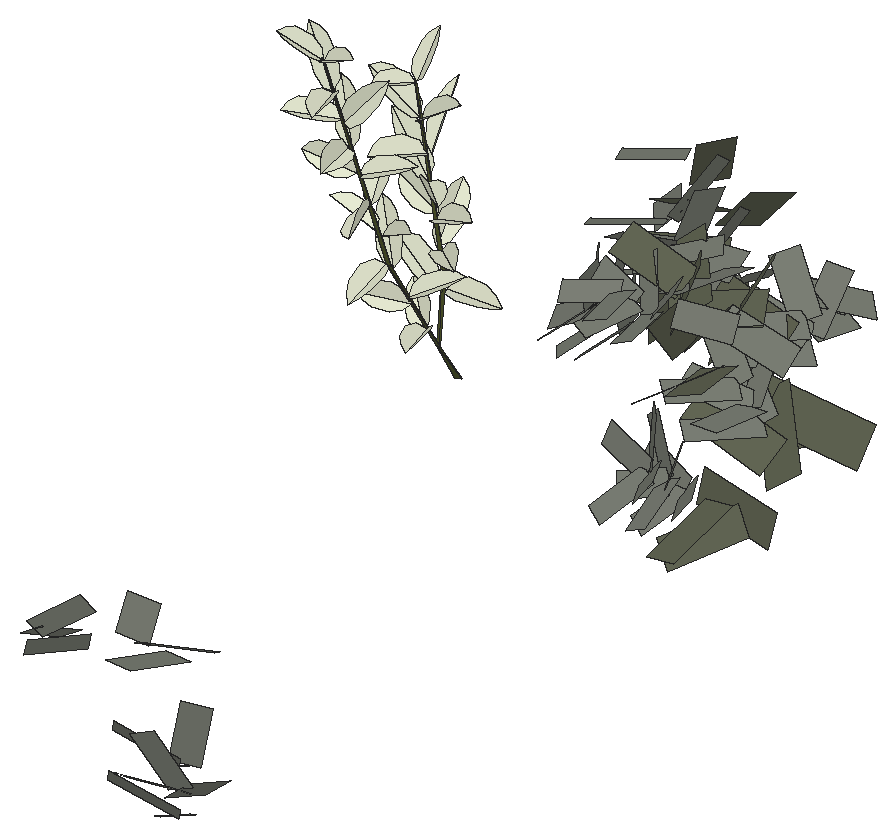
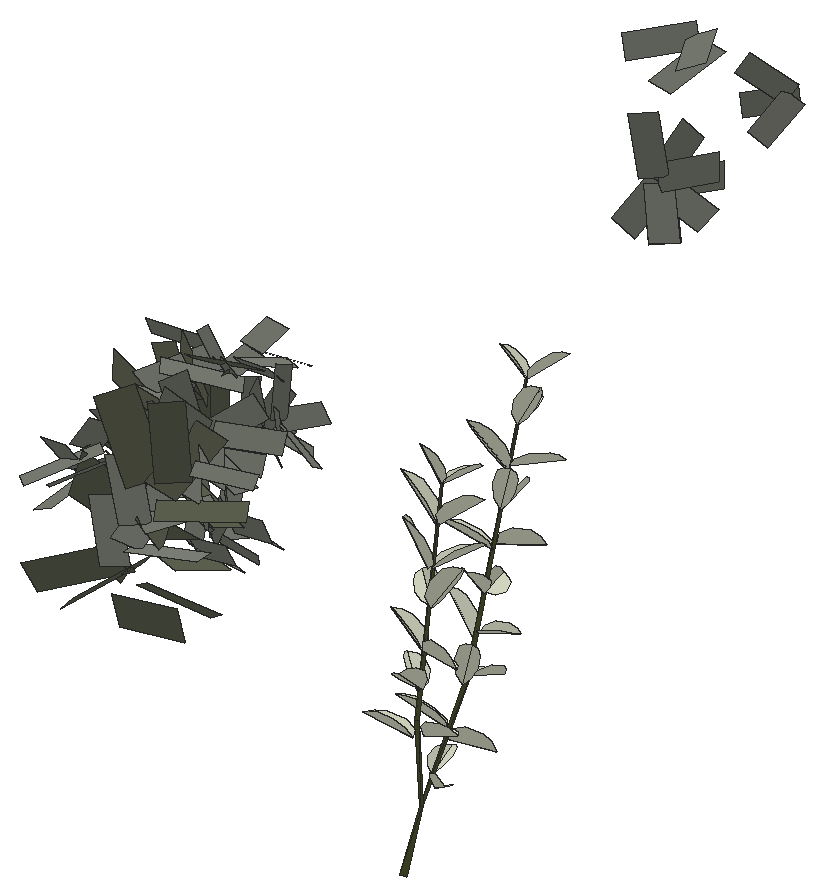
# SketchUp Ruby script. Lengths in inches.
U = 1.inch
M = Sketchup.active_model
def pt(a) = Geom::Point3d.new(a.map { |v| v * U })
def face(e, loops, mat)
  f = e.add_face(loops[0].map { |a| pt(a) })
  loops[1..].each { |l| e.add_face(l.map { |a| pt(a) }).erase! }
  f.material = f.back_material = mat if mat
  f
end
# faces: each face lists its corners as indices into pts; further lists are holes
def faces(e, pts, list, mat = nil) = list.each { |f| face(e, (f[0].is_a?(Array) ? f : [f]).map { |l| l.map { |i| pts[i] } }, mat) }
# xy, xz, yz: faces in a plane at the given z, y or x. An outline is a flat list of corners, or four numbers for a rectangle; further outlines are holes
def ring(l) = l.size == 4 ? [[l[0], l[1]], [l[2], l[1]], [l[2], l[3]], [l[0], l[3]]] : l.each_slice(2).to_a
def flat(e, list, mat, &to3) = list.each { |f| face(e, (f[0].is_a?(Array) ? f : [f]).map { |l| ring(l).map { |u, v| to3.(u, v) } }, mat) }
def xy(e, z, list, mat = nil) = flat(e, list, mat) { |x, y| [x, y, z] }
def xz(e, y, list, mat = nil) = flat(e, list, mat) { |x, z| [x, y, z] }
def yz(e, x, list, mat = nil) = flat(e, list, mat) { |y, z| [x, y, z] }
def lines(e, pts, list) = list.each { |a, b| e.add_line(pt(pts[a]), pt(pts[b])) }
# prism: a flat outline (further loops are holes) pulled along v
def prism(e, loops, v, mat = nil)
  f = face(e, loops, mat); d = Geom::Vector3d.new(v.map { |x| x * U })
  f.pushpull(f.normal.samedirection?(d) ? d.length : -d.length)
end
def box(e, o, s, mat = nil) = prism(e, [[o, [o[0] + s[0], o[1], o[2]], [o[0] + s[0], o[1] + s[1], o[2]], [o[0], o[1] + s[1], o[2]]]], [0, 0, s[2]], mat)
def at(x, y, z, deg = 0) = Geom::Transformation.translation(pt([x, y, z])) * Geom::Transformation.rotation(ORIGIN, Z_AXIS, deg.degrees)
def axes(o, x, y, z) = Geom::Transformation.new([*x, 0, *y, 0, *z, 0, *pt(o).to_a, 1])
def part(name) = M.definitions.add(name)
# library, detail: a bought-in or finely detailed component or shape, given as its bounding box
def library(name, o, s) = part(name).tap { |d| box(d.entities, o, s) }
def detail(e, o, s) = box(e.add_group.entities, o, s)
def put(e, d, t, mat = nil) = e.add_instance(d, t).tap { |i| i.material = mat if mat }
def group(e, t, mat = nil) = e.add_group.tap { |g| g.transformation = t; g.material = mat if mat }.entities
root = M.entities
M.materials.add("asdfasdf0165f6asdLeafVar1sfd015as60f1as6").color = [231, 235, 211]
M.materials.add("dw_stemssadfasdfa0sdf1s01d6w1").color = [90, 97, 50]
M.materials.add("viburnumblaasdfas0df1w06d").color = [98, 102, 84]
M.materials.add("viburnumbladsadfasdfad0w122").color = [125, 129, 119]
c1 = part("vdw_leaf\#3")
p = [[0,0,0],[-2.77,1.61,2.32],[-4.3125,6.1,4.5],[-3.97,13.49,6.09],[-2.47,18.57,6.3],[-0.2,22.73,5.75],
  [2.54,19.66,6.85],[4.3,15.93,7.09],[5.03,7.6,5.43],[3.32,1.76,2.74]]
faces(c1.entities,p,[[0,1,2,3,4,5],[0,5,6,7,8,9]],"asdfasdf0165f6asdLeafVar1sfd015as60f1as6")
c2 = part("dw_brancj_2\#2")
p = [[9.7,-0.22,29.95],[0.23,-1.96,0.34],[-0.05,1.51,0.11],[9.65,1.51,29.46],[18.64,-8.75,84.43],[18.96,-6.63,84.625],
  [1.53,6.02,63.68],[1.42,8.18,63.25],[-10.58,8.77,161.17],[-10.41,9.98,160.68],[26.34,-9.37,211.72],[26.57,-8.28,211.23]]
faces(c2.entities,p,[[0,1,2],[0,2,3],[4,0,3],[4,3,5],[6,0,3],[6,3,7],[8,6,7],[8,7,9],
  [10,4,5],[10,5,11]],"dw_stemssadfasdfa0sdf1s01d6w1")
c3 = part("vdw_branch2\#3")
put(c3.entities,c1,axes([19.53,-5.9,102.42],[1.12377,-0.50004,0],[0.46097,1.03596,0.47664],[-0.19377,-0.43548,1.13389]))
put(c3.entities,c1,axes([-5.89,6.52,109.44],[-1.07209,0.83679,0],[-0.77141,-0.98832,0.52702],[0.32427,0.41545,1.25373]))
put(c3.entities,c1,axes([-0.44,8.23,75.28],[0.88709,-0.9947,0],[0.92159,0.82189,0.33087],[-0.25219,-0.22491,1.26111]))
put(c3.entities,c1,axes([24.71,-8.97,190.81],[-0.82641,0.91101,0],[-0.83983,-0.76184,0.47664],[0.35303,0.32025,1.13389]))
put(c3.entities,c1,axes([-2.29,8.24,91.35],[1.24603,-0.47303,0],[0.43826,1.15445,0.33087],[-0.11993,-0.31592,1.26111]))
put(c3.entities,c1,axes([12.26,-3.11,37.92],[-0.64625,1.02205,0.22511],[-1.04383,-0.61044,-0.22511],[-0.07533,-0.30931,1.18809]))
put(c3.entities,c1,axes([26.17,-9.17,210.27],[-0.99452,-0.10453,0],[0.09636,-0.91681,0.38752],[-0.04051,0.38539,0.92186]))
put(c3.entities,c1,axes([-6.07,9.4,125.35],[-0.90214,-0.98107,0],[0.90896,-0.83583,0.33087],[-0.24874,0.22873,1.26111]))
put(c3.entities,c1,axes([-4.13,7.29,110.58],[0.44715,-1.078,0.64369],[1.05816,0.63649,0.33087],[-0.58725,0.40856,1.09216]))
put(c3.entities,c1,axes([23.91,-8.22,171.96],[0.62307,0.85009,-0.63406],[-0.71531,0.8798,0.47664],[0.78296,0.12729,0.94004]))
put(c3.entities,c2,at(-0.09,0.18,-0.25),"dw_stemssadfasdfa0sdf1s01d6w1")
put(c3.entities,c1,axes([23.34,-9.65,156.59],[-0.31364,-1.00782,0.58216],[1.10369,-0.17062,0.29925],[-0.17137,0.6239,0.98776]))
put(c3.entities,c1,axes([15.03,-3.37,58.83],[-1.05425,-0.00194,0.58442],[-0.14303,-1.11707,-0.26172],[0.55355,-0.3046,0.99755]))
put(c3.entities,c1,axes([-11.625,9.46,160.37],[0.36812,0.92978,0],[-0.85713,0.33936,0.38752],[0.3603,-0.14265,0.92186]))
put(c3.entities,c1,axes([21.32,-8.53,138.72],[1.21379,0.19904,0],[-0.19904,1.21379,0],[0,0,1.23]))
put(c3.entities,c1,axes([22.54,-9.2,141.43],[-1.02887,0.17955,0.60182],[-0.23387,-1.13057,-0.06253],[0.56696,-0.17376,1.02111]))
put(c3.entities,c1,axes([23.9,-8.82,173.84],[-1.14567,-0.37474,0],[0.35918,-1.0981,0.04438],[-0.01409,0.04308,1.17993]))
put(c3.entities,c1,axes([-7.84,8.92,143.59],[-1.26971,0.40522,0],[-0.37543,-1.17638,0.33087],[0.10274,0.32192,1.26111]))
put(c3.entities,c1,axes([19.77,-8.01,85.98],[-0.32405,-1.14591,0.18674],[1.10278,-0.32969,-0.10948],[0.15845,0.14442,1.16117]))
put(c3.entities,c1,axes([-0.62,5.76,76.34],[-0.08879,1.17576,-0.67771],[-1.34525,-0.16582,-0.11144],[-0.17897,0.66309,1.17383]))
put(c3.entities,c1,axes([20.49,-8.22,121.07],[0.39924,-0.78471,-0.8233],[1.08735,0.33121,0.2116],[0.09035,-0.83005,0.83495]))
put(c3.entities,c1,axes([15.15,-3.72,62.9],[1.16251,0.40128,-0.0211],[-0.39924,1.16074,0.07874],[0.0456,-0.06757,1.2273]))
put(c3.entities,c1,axes([20.72,-8.08,120.26],[-0.03693,1.2277,-0.06551],[-1.22944,-0.03698,0],[-0.00197,0.06548,1.22825]))
put(c3.entities,c1,axes([22.58,-8.36,155.57],[-0.56247,1.09386,0],[-1.00839,-0.51852,0.47664],[0.42389,0.21796,1.13389]))
put(c3.entities,c1,axes([3.97,3.13,57.96],[-1.09459,0.76041,0],[-0.72262,-1.0402,-0.1735],[-0.10109,-0.14552,1.29352]))
put(c3.entities,c1,axes([-10.8,9.06,160.75],[-0.66334,-0.72138,0],[0.66835,-0.61458,0.24329],[-0.1829,0.16818,0.92729]))
put(c3.entities,c1,axes([19.06,-9.3125,103.96],[-1.01345,0.25553,-0.60051],[-0.2265,-1.12952,-0.09839],[-0.59598,0.03076,1.01889]))
put(c3.entities,c1,axes([18.07,-6.2,81.7],[-0.56247,1.09386,0],[-1.00839,-0.51852,0.47664],[0.42389,0.21796,1.13389]))
put(c3.entities,c1,axes([12.95,-0.39,43.31],[0.13044,-1.19832,0],[1.11025,0.12085,0.29925],[-0.30382,-0.03307,1.14057]))
put(c3.entities,c1,axes([2.28,8.28,56.18],[1.32413,-0.31027,0],[0.30923,1.31968,-0.11144],[0.02542,0.1085,1.35543]))
put(c3.entities,c1,axes([-7.55,9.96,143.07],[1.34251,-0.21744,0],[0.20045,1.23761,0.52702],[-0.08426,-0.52024,1.25373]))
put(c3.entities,c1,axes([26.15,-8.25,210.66],[0.94661,-0.25364,0],[0.235,0.87703,0.24329],[-0.06431,-0.24,0.92729]))
put(c3.entities,c1,axes([-6.48,11.37,125.16],[0.64635,1.10315,0.46356],[-1.16569,0.46153,0.52702],[0.27017,-0.6478,1.16488]))
put(c3.entities,c1,axes([25.74,-8.35,191.28],[0.13044,-1.19832,0],[1.11025,0.12085,0.29925],[-0.30382,-0.03307,1.14057]))
put(c3.entities,c1,axes([-5.125,7.47,91.6],[-1.10024,0.63688,0.48318],[-0.78682,-1.00808,-0.46292],[0.14137,-0.65404,1.184]))
c4 = part("Component\#315")
p = [[0.25,0,0],[2.05,0.01,0.35],[1.81,4.2,1.66],[0,4.19,1.3125]]
faces(c4.entities,p,[[0,1,2,3]],"viburnumbladsadfasdfad0w122")
c5 = part("viburnumblad2")
put(c5.entities,c4,axes([-19.23,-4.49,-32.18],[83.35428,0,0],[0,79.38502,0],[0,0,83.35428]))
c6 = part("Component\#314")
p = [[0.14,0,0],[2.58,0.05,0.25],[2.44,5.11,2.64],[0,5.05,2.39]]
faces(c6.entities,p,[[0,1,2,3]],"viburnumblaasdfas0df1w06d")
c7 = part("viburnumblad1\#2")
put(c7.entities,c6,axes([-37.25,6.23,19.31],[75.98784,0,0],[0,65.50676,0],[0,0,75.98784]))
put(root,c3,axes([2173.54,345.22,7.57],[0.0254,-0.1143,-0.07152],[0.12761,0.02836,0],[0.01261,-0.05674,0.14408]))
put(root,c5,axes([2192.125,342.61,30.04],[-0.00355,0.00962,-0.00319],[-0.00963,-0.00512,-0.00451],[-0.00533,0.00188,0.0087]))
put(root,c5,axes([2195.05,336.95,29.38],[-0.00445,0.01048,-0.00645],[-0.00976,-0.00718,-0.00494],[-0.00749,0.00313,0.01026]))
put(root,c7,axes([2196.33,341.9,24.84],[-0.00719,0.01195,-0.00129],[-0.01278,-0.0083,-0.00564],[-0.00429,-0.00131,0.01125]))
put(root,c5,axes([2193.95,337.49,28.26],[0.00877,0.00751,0.00615],[-0.00546,0.01067,-0.00523],[-0.00802,0.00094,0.01029]))
put(root,c5,axes([2194.91,329.84,25.875],[-0.00095,0.00927,0.00479],[-0.00714,0.003,-0.00705],[-0.00723,-0.00378,0.00515]))
put(root,c5,axes([2195.66,336.75,27.67],[0.00306,0.01272,-0.00021],[-0.01084,0.00248,-0.00806],[-0.00742,0.00196,0.01059]))
put(root,c5,axes([2194.36,331.05,25.81],[0.0062,-0.00344,0.00762],[-0.00192,0.00879,0.00527],[-0.00787,-0.00449,0.00364]))
put(root,c7,axes([2193.96,344.27,28.05],[-0.00729,-0.01049,-0.00199],[0.00959,-0.00792,0.00787],[-0.00649,0.00328,0.00895]))
put(root,c7,axes([2195.66,343.26,26.96],[-0.01203,-0.00093,-0.00471],[0.00029,-0.01476,0.00205],[-0.00435,0.00215,0.01023]))
put(root,c5,axes([2195.62,330.71,25.125],[0.00371,0.00412,0.00878],[-0.006,0.0085,-0.00147],[-0.00737,-0.00446,0.00446]))
put(root,c5,axes([2195.48,330.16,27.01],[-0.0062,0.00344,-0.00762],[-0.00004,-0.00961,-0.00424],[-0.0081,-0.00223,0.0048]))
put(root,c5,axes([2193.96,279.43,27.12],[0.00984,0.00064,0.00419],[0.00246,0.0079,-0.00679],[-0.00344,0.00689,0.00616]))
put(root,c5,axes([2197.32,336.78,26.98],[-0.00427,0.01006,-0.00619],[-0.01054,-0.00775,-0.00533],[-0.00749,0.00313,0.01026]))
put(root,c5,axes([2196.43,330.1,26],[-0.00506,0.00898,-0.002],[-0.00471,-0.00455,-0.00828],[-0.00753,-0.00286,0.00529]))
put(root,c5,axes([2196.67,337.5,28.44],[-0.00935,0.0021,-0.00891],[-0.00409,-0.01235,0.00138],[-0.00819,0.00377,0.00948]))
put(root,c5,axes([2197.66,341.57,21.89],[-0.00305,0.01398,0.00068],[-0.01364,-0.00282,-0.0033],[-0.00279,-0.00128,0.01326]))
put(root,c5,axes([2194.93,331.37,26.95],[0.00095,-0.00927,-0.00479],[0.00517,-0.00382,0.00808],[-0.00874,-0.00294,0.00329]))
put(root,c7,axes([2198.51,336.08,23.77],[0.00387,0.01311,0.00437],[-0.0121,0.00667,-0.00928],[-0.00906,-0.00102,0.01108]))
put(root,c5,axes([2197.77,341.67,23.78],[-0.01149,0.00801,-0.00297],[-0.00766,-0.01186,-0.00235],[-0.00352,-0.00017,0.01315]))
put(root,c5,axes([2196.13,337.19,25.88],[0.00916,0.00784,0.00642],[-0.00492,0.00961,-0.00471],[-0.00802,0.00094,0.01029]))
put(root,c5,axes([2195.07,337.91,26.84],[0.00935,-0.0021,0.00891],[0.00182,0.01184,0.00088],[-0.00893,0.00067,0.00953]))
put(root,c5,axes([2194.54,339.03,28.43],[0.00445,-0.01048,0.00645],[0.00766,0.00772,0.00727],[-0.00963,0.0013,0.00876]))
put(root,c5,axes([2195.59,331.73,25.73],[0.00506,-0.00898,0.002],[0.00284,0.00386,0.00969],[-0.00844,-0.00386,0.00315]))
put(root,c5,axes([2196.53,331.62,24.8],[0.00595,-0.0033,0.00732],[-0.00208,0.00949,0.0057],[-0.00787,-0.00449,0.00364]))
put(root,c5,axes([2194.78,278.79,26.22],[0.00494,-0.0045,0.00826],[0.00853,0.00632,-0.00167],[-0.00419,0.00708,0.00554]))
put(root,c5,axes([2196.32,331.42,26.66],[-0.00371,-0.00412,-0.00878],[0.00371,-0.00856,0.0023],[-0.0086,-0.00227,0.00398]))
put(root,c5,axes([2195.18,280.01,27],[-0.00286,-0.007,0.00749],[0.00939,0.00159,0.0048],[-0.00429,0.00766,0.00474]))
put(root,c5,axes([2197.46,330.99,26.08],[-0.00487,0.00336,-0.00745],[-0.00004,-0.00961,-0.00424],[-0.00872,-0.00185,0.00395]))
put(root,c5,axes([2198.91,327.91,29.23],[-0.00345,0.00905,0.004],[-0.00954,-0.00184,-0.00399],[-0.00252,-0.00485,0.0079]))
put(root,c5,axes([2196.28,338.97,27.74],[-0.00306,-0.01272,0.00021],[0.00831,-0.00183,0.01011],[-0.0097,0.00247,0.00842]))
put(root,c5,axes([2198.84,328.77,28.19],[0.00404,0.00727,0.00631],[-0.0093,0.00487,0.00025],[-0.00255,-0.00567,0.00738]))
put(root,c5,axes([2197.03,332.03,25.95],[0.00099,-0.00968,-0.005],[0.00466,-0.00344,0.00728],[-0.00874,-0.00294,0.00329]))
put(root,c5,axes([2196.52,338.54,26.05],[0.00502,-0.00971,0.00503],[0.00766,0.00772,0.00727],[-0.00909,0.00016,0.0094]))
put(root,c5,axes([2199.24,329.58,16.625],[0.00409,0.00375,0.00971],[-0.00938,0.00585,0.00169],[-0.00452,-0.00876,0.00528]))
put(root,c7,axes([2199.37,336.62,21.3],[0.00862,0.00382,0.01082],[-0.00301,0.01604,-0.00327],[-0.01117,-0.00026,0.009]))
put(root,c5,axes([2198.79,342.91,22.4375],[-0.0132,-0.00264,-0.00489],[0.00251,-0.01421,0.00089],[-0.00477,0.0001,0.01275]))
put(root,c7,axes([2196.78,343.4,26.34],[-0.0079,-0.01248,0.00117],[0.01398,-0.00821,0.00596],[-0.0035,0.004,0.01323]))
put(root,c7,axes([2198.75,333.08,24.51],[0.00244,-0.01122,0.00057],[0.00459,0.00184,0.0121],[-0.01018,-0.00173,0.00319]))
put(root,c7,axes([2201.18,331.21,28.69],[0.00232,0.01057,0.00577],[-0.01348,0.00407,-0.00203],[-0.00316,-0.00514,0.01068]))
put(root,c5,axes([2200.07,328.75,28.74],[-0.00892,0.00552,-0.00065],[-0.0045,-0.00791,-0.00542],[-0.00314,-0.00411,0.00807]))
put(root,c5,axes([2197.68,343.47,23.97],[-0.00718,-0.01175,-0.00394],[0.01087,-0.00815,0.00451],[-0.0058,-0.00063,0.01231]))
put(root,c5,axes([2199.07,329.84,27.46],[0.0088,0.00119,0.00472],[-0.00418,0.00904,0.00526],[-0.00322,-0.0061,0.00681]))
put(root,c5,axes([2200.45,329.14,17.23],[-0.00876,0.00688,0.00103],[-0.00474,-0.00469,-0.00897],[-0.00509,-0.00746,0.00659]))
put(root,c5,axes([2200.76,330.16,16.05],[-0.0033,0.00751,0.0076],[-0.0089,0.00112,-0.00498],[-0.00448,-0.00819,0.00616]))
put(root,c5,axes([2201.45,334.27,30.71],[-0.00774,0.01238,-0.00167],[-0.01057,-0.00772,-0.00819],[-0.0074,-0.00296,0.01235]))
put(root,c5,axes([2200.6,331.42,15.23],[0.00419,0.0043,0.00836],[-0.00938,0.00585,0.00169],[-0.00405,-0.0083,0.0063]))
put(root,c5,axes([2199.51,331.1,16.22],[0.00908,-0.00221,0.00614],[-0.004,0.00655,0.00828],[-0.00518,-0.00884,0.00448]))
put(root,c5,axes([2199.6,328.7,30.03],[-0.00916,-0.00124,-0.00492],[0.00298,-0.00959,-0.00307],[-0.00406,-0.0039,0.00779]))
put(root,c5,axes([2201.47,334.76,28.64],[0.00099,0.01426,0.00559],[-0.01157,0.00302,-0.00566],[-0.00706,-0.00428,0.01216]))
put(root,c7,axes([2200.93,332.31,26.7],[0.00961,0.00314,0.00694],[-0.00599,0.01265,0.00258],[-0.0056,-0.00466,0.00986]))
put(root,c5,axes([2198.74,343.99,20.93],[-0.00599,-0.01069,-0.00483],[0.01087,-0.00815,0.00451],[-0.00654,-0.00189,0.01181]))
put(root,c5,axes([2199.03,330.46,17.7],[0.00876,-0.00688,-0.00103],[0.00337,0.00275,0.0103],[-0.00608,-0.00838,0.00422]))
put(root,c5,axes([2201.66,331.15,15.75],[-0.00914,0.00718,0.00108],[-0.00427,-0.00422,-0.00808],[-0.00509,-0.00746,0.00659]))
put(root,c5,axes([2200.54,329.96,28.33],[-0.00798,-0.00075,-0.00527],[0.00298,-0.00959,-0.00307],[-0.00502,-0.00401,0.00721]))
put(root,c7,axes([2204.23,335.5,26.16],[-0.0074,0.01393,0.00333],[-0.01491,-0.00558,-0.00981],[-0.00631,-0.00654,0.01332]))
put(root,c7,axes([2200.77,333.52,24.66],[-0.00329,-0.00864,-0.00687],[0.00632,-0.00867,0.00771],[-0.00921,-0.00096,0.00528]))
put(root,c5,axes([2201.15,330.65,17.21],[-0.00908,0.00221,-0.00614],[0.00272,-0.00885,-0.00722],[-0.00599,-0.007,0.00633]))
put(root,c7,axes([2200.12,331.92,26.2],[0.00733,-0.00886,0.00054],[0.00689,0.00642,0.00923],[-0.00652,-0.00466,0.00706]))
put(root,c5,axes([2199.67,330.6875,28.29],[0.0036,-0.00945,-0.00418],[0.00778,0.00056,0.0052],[-0.00475,-0.00515,0.0067]))
put(root,c5,axes([2200.23,330.03,18.3],[-0.00409,-0.00375,-0.00971],[0.008,-0.0078,-0.00036],[-0.00665,-0.00708,0.00553]))
put(root,c7,axes([2204.46,336.27,23.27],[0.00378,0.01126,0.01091],[-0.0152,0.00977,-0.00482],[-0.0086,-0.00789,0.01113]))
put(root,c5,axes([2201.49,279.06,30.08],[0.01014,0.00518,-0.00703],[-0.00774,0.0103,-0.00358],[0.00402,0.00678,0.0108]))
put(root,c5,axes([2203.37,282.3125,20.93],[-0.00504,0.005,-0.01036],[-0.01063,-0.00635,0.00211],[-0.0044,0.00962,0.00678]))
put(root,c7,axes([2204.01,336.25,11.11],[0.00278,0.00293,0.01264],[-0.01346,0.00734,0.00126],[-0.00579,-0.01128,0.00389]))
put(root,c5,axes([2202.73,335.52,29.79],[-0.01142,0.0037,-0.00741],[-0.00214,-0.01514,-0.00425],[-0.0084,-0.00214,0.01187]))
put(root,c7,axes([2204.05,334.18,12.875],[-0.00836,0.0066,0.00609],[-0.00962,-0.00288,-0.01008],[-0.00344,-0.01004,0.00615]))
put(root,c5,axes([2202.46,333.38,22.25],[0.00865,0.00796,0.00491],[-0.00918,0.00854,0.00232],[-0.00184,-0.00511,0.01153]))
put(root,c5,axes([2203.73,333.5625,20.85],[-0.00016,0.01206,0.00411],[-0.0133,0.00032,-0.00146],[-0.00141,-0.0041,0.01199]))
put(root,c5,axes([2200.19,331.44,17.43],[0.0033,-0.00751,-0.0076],[0.00833,-0.00317,0.00675],[-0.00669,-0.00765,0.00466]))
put(root,c7,axes([2204.34,335.17,16.42],[0.00263,0.01141,0.00764],[-0.01577,0.00377,-0.0002],[-0.00192,-0.0074,0.01171]))
put(root,c7,axes([2203.01,333.01,23.87],[-0.00905,0.00252,-0.00817],[0.0005,-0.01365,-0.00475],[-0.00803,-0.00297,0.00749]))
put(root,c5,axes([2202.12,282.28,19.95],[0.01002,0.00748,-0.00127],[-0.0057,0.00603,-0.00944],[-0.00501,0.0081,0.0082]))
put(root,c5,axes([2203.53,281.07,19.7],[0.00352,0.00882,-0.00823],[-0.01182,-0.0007,-0.00581],[-0.00432,0.00892,0.00772]))
put(root,c7,axes([2203.13,342.67,15.03],[-0.01009,0.00576,0.00864],[-0.00958,-0.01423,-0.00203],[0.00708,-0.00619,0.01118]))
put(root,c5,axes([2204.01,333.03,22.52],[-0.00888,0.0091,0.0009],[-0.00895,-0.0084,-0.00345],[-0.00187,-0.00303,0.01224]))
put(root,c7,axes([2201.71,337.72,19.45],[0.00372,-0.01109,0.0102],[0.00971,0.0119,0.0094],[-0.01253,0.00356,0.00844]))
put(root,c7,axes([2203.31,333.33,14.86],[-0.01158,0.00263,-0.00305],[0.00041,-0.00999,-0.01013],[-0.00401,-0.00833,0.00806]))
put(root,c5,axes([2201.36,332.1,16.76],[-0.00392,-0.0036,-0.00932],[0.00864,-0.00842,-0.00039],[-0.00665,-0.00708,0.00553]))
put(root,c5,axes([2204.02,338.46,23.2],[-0.00038,0.01114,0.00561],[-0.01176,-0.00241,0.0034],[0.00455,-0.00528,0.01006]))
put(root,c5,axes([2203.17,334.625,19.44],[0.00904,0.00831,0.00513],[-0.00826,0.00768,0.00209],[-0.00184,-0.00511,0.01153]))
put(root,c5,axes([2201.15,278.58,28.31],[0.01295,-0.00298,-0.00152],[0.00183,0.01176,-0.00745],[0.00286,0.00667,0.01124]))
put(root,c5,axes([2204.24,342.42,24.03],[-0.00577,0.00885,0.00437],[-0.00922,-0.00664,0.00128],[0.00353,-0.00288,0.01049]))
put(root,c5,axes([2204.75,334.41,19.71],[-0.00853,0.00873,0.00086],[-0.00967,-0.00907,-0.00372],[-0.00187,-0.00303,0.01224]))
put(root,c5,axes([2204.91,280.39,18.93],[-0.00484,0.0048,-0.00995],[-0.01148,-0.00686,0.00228],[-0.0044,0.00962,0.00678]))
put(root,c7,axes([2203.74,336.64,14.36],[0.01152,0.00345,0.00714],[-0.0073,0.01349,0.00527],[-0.00481,-0.00695,0.01113]))
put(root,c5,axes([2204.5,339.49,22.03],[-0.00848,0.00652,0.00394],[-0.00785,-0.00971,-0.00119],[0.00311,-0.00363,0.01115]))
put(root,c5,axes([2203.61,338.2,24.9375],[0.00829,0.0091,0.00248],[-0.00839,0.00593,0.00669],[0.00415,-0.0063,0.00965]))
put(root,c7,axes([2201.64,333.125,25.51],[-0.001,-0.01064,-0.00433],[0.01169,-0.00333,0.00541],[-0.00539,-0.00308,0.00855]))
put(root,c7,axes([2201.95,334.11,24.94],[0.00803,-0.00983,0.00384],[0.00868,0.0101,0.00771],[-0.00745,-0.00186,0.01082]))
put(root,c5,axes([2204.69,281.88,19.68],[-0.01065,-0.00175,-0.00643],[-0.00418,-0.00769,0.00902],[-0.00519,0.00978,0.00593]))
put(root,c5,axes([2202.61,334.56,20.89],[0.0124,-0.0008,0.00284],[-0.00048,0.01054,0.00506],[-0.0029,-0.00547,0.01114]))
put(root,c5,axes([2203.58,280.29,18.05],[0.01046,0.00781,-0.00132],[-0.00513,0.00543,-0.00849],[-0.00501,0.0081,0.0082]))
put(root,c7,axes([2203.45,333.34,23.95],[-0.01126,-0.00328,-0.00424],[0.0051,-0.0131,-0.00341],[-0.00278,-0.00386,0.0103]))
put(root,c5,axes([2205.125,338.17,24.55],[-0.00883,0.00666,0.00546],[-0.00785,-0.00971,-0.00119],[0.00409,-0.00438,0.01062]))
put(root,c7,axes([2206.37,341.58,14.89],[0.00192,0.00886,0.01301],[-0.01818,-0.00012,0.00276],[0.00142,-0.01315,0.00875]))
put(root,c5,axes([2204.56,343.59,22.76],[-0.01085,0.00184,0.00308],[-0.00218,-0.01013,-0.00164],[0.00269,-0.00234,0.01086]))
put(root,c5,axes([2202.85,281.58,18.49],[0.01065,0.00175,0.00643],[0.00257,0.00902,-0.00671],[-0.00605,0.00763,0.00794]))
put(root,c5,axes([2206.22,342.84,24.4],[-0.01077,0.01075,0.00083],[-0.01084,-0.01091,0.00051],[0.00094,-0.00022,0.01521]))
put(root,c5,axes([2204.78,334.36,21.42],[-0.0124,0.0008,-0.00284],[-0.0002,-0.01247,-0.00265],[-0.00294,-0.00253,0.01214]))
put(root,c5,axes([2204.04,283.45,20.04],[-0.01002,-0.00748,0.00127],[0.00432,-0.00389,0.01114],[-0.00624,0.00932,0.00567]))
put(root,c5,axes([2203.06,339.48,23.95],[0.01211,0.00173,-0.00211],[0,0.01038,0.00684],[0.00312,-0.00685,0.00964]))
put(root,c5,axes([2206.07,334.13,24.06],[0.00252,0.00942,0.00914],[-0.01307,0.00092,0.00265],[0.00124,-0.00944,0.00938]))
put(root,c5,axes([2201.94,280.28,29],[0.00818,-0.0094,0.00487],[0.01043,0.00611,-0.00572],[0.00179,0.0073,0.01107]))
put(root,c5,axes([2206.24,329.16,28.43],[-0.00034,0.00733,0.00907],[-0.01154,0.00172,-0.00184],[-0.00225,-0.00876,0.00608]))
